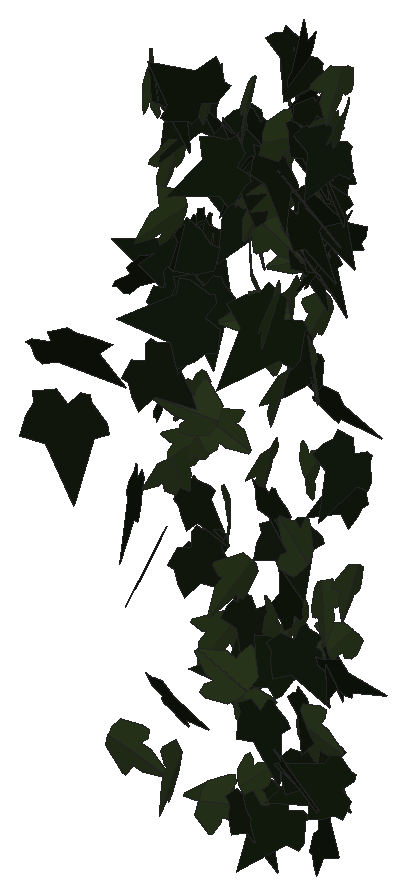
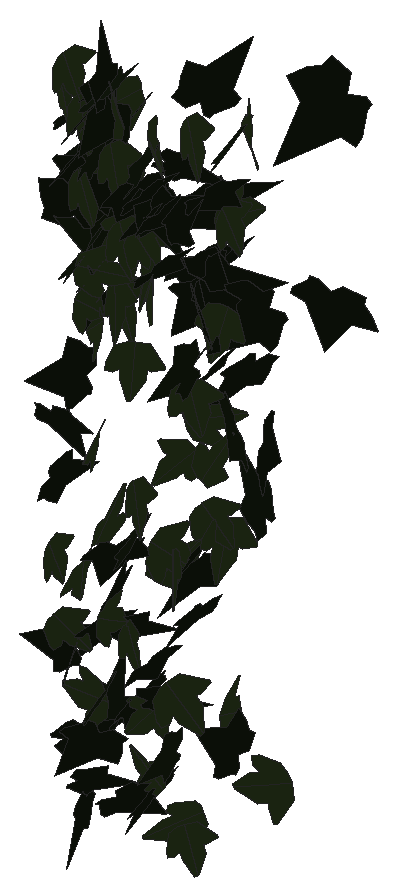
# SketchUp Ruby script. Lengths in inches.
U = 1.inch
M = Sketchup.active_model
def pt(a) = Geom::Point3d.new(a.map { |v| v * U })
def face(e, loops, mat)
  f = e.add_face(loops[0].map { |a| pt(a) })
  loops[1..].each { |l| e.add_face(l.map { |a| pt(a) }).erase! }
  f.material = f.back_material = mat if mat
  f
end
# faces: each face lists its corners as indices into pts; further lists are holes
def faces(e, pts, list, mat = nil) = list.each { |f| face(e, (f[0].is_a?(Array) ? f : [f]).map { |l| l.map { |i| pts[i] } }, mat) }
# xy, xz, yz: faces in a plane at the given z, y or x. An outline is a flat list of corners, or four numbers for a rectangle; further outlines are holes
def ring(l) = l.size == 4 ? [[l[0], l[1]], [l[2], l[1]], [l[2], l[3]], [l[0], l[3]]] : l.each_slice(2).to_a
def flat(e, list, mat, &to3) = list.each { |f| face(e, (f[0].is_a?(Array) ? f : [f]).map { |l| ring(l).map { |u, v| to3.(u, v) } }, mat) }
def xy(e, z, list, mat = nil) = flat(e, list, mat) { |x, y| [x, y, z] }
def xz(e, y, list, mat = nil) = flat(e, list, mat) { |x, z| [x, y, z] }
def yz(e, x, list, mat = nil) = flat(e, list, mat) { |y, z| [x, y, z] }
def lines(e, pts, list) = list.each { |a, b| e.add_line(pt(pts[a]), pt(pts[b])) }
# prism: a flat outline (further loops are holes) pulled along v
def prism(e, loops, v, mat = nil)
  f = face(e, loops, mat); d = Geom::Vector3d.new(v.map { |x| x * U })
  f.pushpull(f.normal.samedirection?(d) ? d.length : -d.length)
end
def box(e, o, s, mat = nil) = prism(e, [[o, [o[0] + s[0], o[1], o[2]], [o[0] + s[0], o[1] + s[1], o[2]], [o[0], o[1] + s[1], o[2]]]], [0, 0, s[2]], mat)
def at(x, y, z, deg = 0) = Geom::Transformation.translation(pt([x, y, z])) * Geom::Transformation.rotation(ORIGIN, Z_AXIS, deg.degrees)
def axes(o, x, y, z) = Geom::Transformation.new([*x, 0, *y, 0, *z, 0, *pt(o).to_a, 1])
def part(name) = M.definitions.add(name)
# library, detail: a bought-in or finely detailed component or shape, given as its bounding box
def library(name, o, s) = part(name).tap { |d| box(d.entities, o, s) }
def detail(e, o, s) = box(e.add_group.entities, o, s)
def put(e, d, t, mat = nil) = e.add_instance(d, t).tap { |i| i.material = mat if mat }
def group(e, t, mat = nil) = e.add_group.tap { |g| g.transformation = t; g.material = mat if mat }.entities
root = M.entities
M.materials.add("efeu1").color = [18, 25, 13]
M.materials.add("efeu2").color = [43, 57, 29]
c1 = part("ivyleaf_9")
p = [[1.54,2.16,1.25],[1.36,2.04,1.19],[-0.21,0.99,0.68],[-0.71,1.11,0.82],[-0.85,0.86,0.67],[-0.8,0.17,0.21],
  [-0.9,-0.01,0.1],[-0.67,-0.16,-0.02],[-0.08,-0.08,-0.05],[-0.03,-0.6,-0.4],[0.65,-0.88,-0.66],[0.83,-0.6,-0.49],
  [1.29,-0.42,-0.43],[1.8125,-0.07,-0.26],[1.21,0.44,0.15]]
faces(c1.entities,p,[[0,1,2,3,4,5,6,7,8,9,10,11,12,13,14]],"efeu1")
c2 = part("ivyleaf_10")
p = [[0,0.5,-0.03],[-0.0625,2.02,-0.43],[-0.19,2.01,-0.46],[-0.54,1.05,-0.29],[-0.52,0.625,-0.18],[-0.83,0.76,-0.28],
  [-1.16,0.64,-0.33],[-1.15,0.33,-0.24],[-0.77,-0.39,0.02],[-0.3,-0.51,0.16],[0.04,-0.48,0.23],[-0.02,2.01,-0.4375],
  [-0.06,2.01,-0.43],[0.04,-0.49,0.23],[0.67,-0.49,0.14],[1.38,0.36,-0.2],[1.375,0.51,-0.24],[0.81,0.65,-0.19],
  [0.62,0.59,-0.15],[0.6,1.09,-0.28],[0.5,1.23,-0.31]]
faces(c2.entities,p,[[0,1,2,3,4,5,6,7,8,9,10],[11,12,0,13,14,15,16,17,18,19,20]],"efeu2")
put(root,c1,axes([548.11,113.9,235.42],[1.28022,0.60227,0.19081],[0.16815,0.09079,-1.41477],[-0.60898,1.29117,0.01048]))
put(root,c1,axes([544.9,118.74,229.05],[-0.84969,-0.61122,-0.89076],[0.69545,0.55774,-1.04609],[0.82668,-1.09743,-0.03553]))
put(root,c1,axes([549.24,122.18,233.34],[-0.22968,-0.83768,-0.9062],[-0.08009,-0.9097,0.86121],[-1.23146,0.2154,0.11301]))
put(root,c1,axes([545.83,122.21,219.59],[0.02801,1.00742,0.6907],[-0.01978,-0.69042,1.00781],[1.2213,-0.03428,0.00048]))
put(root,c1,axes([545.03,123.13,223.66],[-0.22386,0.10081,-1.19076],[1.02169,-0.61225,-0.24391],[-0.61986,-1.04555,0.02801]))
put(root,c2,axes([549.99,123.5,215.83],[0.35261,0.79349,0.70985],[-0.33312,-0.628,0.86747],[1.01121,-0.48357,0.03824]))
put(root,c2,axes([546.32,124.03,210.43],[0.14476,-0.45523,1.14308],[0.69552,-0.91915,-0.45413],[1.01494,0.69481,0.14817]))
put(root,c2,axes([551.84,123.67,234.42],[0.51811,-1.04399,-0.01718],[-0.00669,0.01586,-1.16548],[1.04411,0.51816,0.00105]))
put(root,c1,axes([551.67,124.37,233.12],[-1.22341,-0.5287,0.1001],[-0.0841,-0.0577,-1.33262],[0.53148,-1.22614,0.01955]))
put(root,c1,axes([546.15,123.8125,232.875],[0.65919,-0.61663,-0.69147],[-0.23733,0.70792,-0.85755],[0.89556,0.64148,0.2817]))
put(root,c2,axes([545.22,125.4,235.57],[0.01015,-0.17762,1.12447],[0.13764,-1.11607,-0.17754],[1.13006,0.13753,0.01153]))
put(root,c2,axes([550.83,125.02,232.86],[0.24225,0.07581,-1.10045],[-1.00258,-0.4547,-0.25203],[-0.45998,1.03098,-0.03024]))
put(root,c1,axes([547.15,124.92,232.75],[-0.03803,-1.10121,-0.27767],[0.04772,0.27604,-1.10124],[1.13468,-0.04852,0.037]))
put(root,c2,axes([551.07,125.25,229.74],[0.24564,-1.1153,0.05987],[0.00144,-0.06099,-1.14197],[1.1169,0.24536,-0.0117]))
put(root,c1,axes([546.33,125.65,241.08],[0.25441,0.1856,1.10471],[-0.97872,-0.51423,0.31179],[0.54491,-1.01028,0.04424]))
put(root,c1,axes([544.4,124.68,228.46],[0.38973,-0.54202,-0.89548],[-0.18105,0.90623,-0.62732],[1.03097,0.36404,0.22835]))
put(root,c2,axes([542.2,125.73,209.32],[-0.48501,0.1138,-1.0983],[1.07896,-0.20608,-0.49782],[-0.23465,-1.18281,-0.01893]))
put(root,c2,axes([547.94,126.48,219.05],[-0.11869,-0.72826,0.86435],[0.02016,-0.87033,-0.73053],[1.13007,-0.06096,0.10381]))
put(root,c1,axes([549.83,126.25,239.08],[0.3045,-1.00657,0.18188],[0.0412,-0.17754,-1.05155],[1.02203,0.30705,-0.0118]))
put(root,c1,axes([545.73,125.98,232.6],[-0.48648,0.13082,1.16642],[-1.14777,0.21109,-0.50238],[-0.24551,-1.24605,0.03736]))
put(root,c2,axes([546.11,126.34,225.85],[0.26765,0.20594,1.03616],[-0.80324,-0.65461,0.33759],[0.68618,-0.84661,-0.00898]))
put(root,c1,axes([547.45,126.52,237.94],[-0.92473,-0.2032,0.46252],[-0.44699,-0.12042,-0.9466],[0.2354,-1.02692,0.01949]))
put(root,c1,axes([550.67,126.76,209.875],[0.89426,-0.66762,-0.15371],[0.14247,-0.066,1.11553],[-0.67011,-0.90497,0.03204]))
put(root,c2,axes([542.82,126.73,240.68],[0.22491,-0.08428,1.21566],[1.06356,-0.5898,-0.23766],[0.59478,1.08652,-0.03472]))
put(root,c1,axes([543.08,125.42,231.91],[0.63882,0.73595,0.6306],[0.39256,0.49405,-0.97426],[-0.8861,0.74944,0.02301]))
put(root,c1,axes([550.96,126.51,236.78],[0.64558,-0.77965,-0.32909],[-0.15457,0.29831,-1.00997],[0.83202,0.66037,0.06771]))
put(root,c1,axes([549.55,127.14,214.9],[-0.63647,-0.29447,0.5931],[-0.48834,-0.34687,-0.69626],[0.44723,-0.79783,0.0838]))
put(root,c1,axes([543.6875,126.87,240.48],[0.47469,-0.9316,0.0422],[0.01647,-0.03897,-1.04556],[0.93241,0.47496,-0.00301]))
put(root,c1,axes([550.82,127.38,229.99],[-0.11433,-0.75041,0.67425],[-0.14082,-0.66005,-0.75848],[0.99895,-0.17893,-0.02976]))
put(root,c1,axes([550.39,126.73,237.89],[0.85433,-0.61914,0.39765],[0.32146,-0.23407,-1.05509],[0.66191,0.91281,-0.00084]))
put(root,c1,axes([544.83,127.24,233.66],[-0.15173,0.10468,-1.0156],[0.63336,-0.79566,-0.17664],[-0.80078,-0.64915,0.05272]))
put(root,c2,axes([549.77,126.18,240.27],[-0.11552,-0.19847,-1.04461],[0.52734,0.90173,-0.22964],[0.92331,-0.53985,0.00046]))
put(root,c1,axes([544.44,127.64,229.32],[-0.09571,-0.90601,0.46397],[0.02556,-0.46801,-0.90862],[1.01758,-0.07346,0.06647]))
put(root,c1,axes([545.39,126.47,219.18],[0.36268,-0.51266,-0.89681],[-0.186,0.90254,-0.59115],[1.01612,0.34819,0.21189]))
put(root,c1,axes([548.39,127.19,212.17],[0.28537,-1.01097,-0.18089],[-0.05662,0.17197,-1.05044],[1.02546,0.29083,-0.00766]))
put(root,c1,axes([543.23,127.26,211.11],[0.49177,-0.46473,0.78965],[0.62213,-0.48859,-0.67498],[0.67267,0.79163,0.04698]))
put(root,c2,axes([543.57,127.42,237.01],[0.04502,-0.94848,0.37058],[0.13585,-0.36203,-0.94311],[1.0092,0.09105,0.11042]))
put(root,c1,axes([544.14,126.21,226.11],[-0.0895,0.57934,1.11363],[-0.18649,1.09793,-0.58616],[-1.24138,-0.20671,0.00777]))
put(root,c1,axes([547.66,127.22,207.77],[0.47472,-0.93415,-0.35024],[-0.13461,0.32435,-1.04754],[0.98853,0.49278,0.02555]))
put(root,c1,axes([550.39,127.49,240.21],[0.48792,-0.87105,-0.11834],[-0.07118,0.09576,-0.99828],[0.87616,0.49285,-0.0152]))
put(root,c2,axes([550.41,127.7,229.7],[-0.47713,0.53739,-0.87193],[0.52184,-0.70014,-0.71707],[-0.88132,-0.70549,0.04747]))
put(root,c1,axes([551.43,128.08,239.78],[-0.3104,-0.90416,0.41479],[-0.04839,-0.42027,-0.95233],[0.99358,-0.30293,0.0832]))
put(root,c1,axes([548.93,128.07,207.33],[-0.70046,-0.81117,0.30777],[-0.18438,-0.24734,-1.07154],[0.84778,-0.72401,0.02124]))
put(root,c1,axes([549.87,127.64,234.5],[0.6541,-0.61005,0.54218],[0.38555,-0.38144,-0.89432],[0.71935,0.75915,-0.01367]))
put(root,c2,axes([547.38,127.57,208.42],[0.57559,-0.17565,-0.67433],[0.64036,-0.21157,0.60171],[-0.27478,-0.86097,-0.01029]))
put(root,c1,axes([544.59,127.36,221.12],[0.52327,-0.6204,-0.48779],[-0.18249,0.4743,-0.79899],[0.76781,0.53554,0.14254]))
put(root,c1,axes([543.99,127.74,231.3],[0.53555,-0.9246,-0.15239],[-0.06095,0.14079,-1.06836],[0.93509,0.53872,0.01765]))
put(root,c2,axes([545.32,127.71,240.76],[0.14923,-1.08152,-0.05502],[-0.00686,0.05459,-1.09177],[1.0829,0.14939,0.00066]))
put(root,c1,axes([544.5,127.57,233.1],[-0.271,-0.50327,-0.93319],[0.51722,0.77806,-0.56981],[0.92553,-0.58216,0.04518]))
put(root,c1,axes([551.67,128.23,209.31],[-0.39258,-0.77052,-0.50341],[-0.21501,-0.45537,0.86467],[-0.89492,0.44741,0.01309]))
put(root,c2,axes([545.73,127.2,207.08],[-0.14319,-0.3257,-1.00644],[0.76737,0.66708,-0.32506],[0.72812,-0.76709,0.14465]))
put(root,c2,axes([543.67,127.65,232.23],[-1.01831,0.00515,-0.09705],[0.09704,-0.00231,-1.01832],[-0.00535,-1.02292,0.00181]))
put(root,c2,axes([549.79,128,219.84],[-0.24524,1.02137,0.39064],[0.06949,-0.38497,1.0502],[1.09132,0.25404,0.02091]))
put(root,c2,axes([543.89,128.45,225.13],[-0.20392,-0.51942,-0.76545],[-0.30548,-0.70205,0.55778],[-0.87315,0.36693,-0.01637]))
put(root,c2,axes([543.41,127.68,222.04],[-0.40268,-0.98545,-0.34394],[0.12908,0.3188,-1.06455],[1.03573,-0.42286,-0.00104]))
put(root,c2,axes([550.1,128.12,211.75],[-0.16467,0.10605,-1.11198],[1.00427,-0.47807,-0.19431],[-0.48907,-1.01739,-0.02461]))
put(root,c2,axes([548.55,127.68,234.85],[-0.67035,-0.33147,-0.64256],[0.62083,0.18523,-0.74323],[0.37058,-0.90991,0.08278]))
put(root,c2,axes([547.25,127.83,212.0625],[-0.69725,-0.07575,-0.56826],[0.57195,-0.03088,-0.69767],[0.0391,-0.89896,0.07185]))
put(root,c1,axes([550.34,128.47,237.6],[0.69213,-0.80626,0.01305],[0.00159,0.01856,1.06251],[-0.80636,-0.692,0.01329]))
put(root,c2,axes([545.71,127.45,224.75],[0.47264,0.38009,0.74129],[0.39346,0.64938,-0.58383],[-0.73428,0.59262,0.16431]))
put(root,c2,axes([547.8125,127.4,232.76],[-0.5379,0.34428,0.90384],[-0.75066,0.50355,-0.63855],[-0.60989,-0.92342,-0.01122]))
put(root,c1,axes([549.57,127.96,215.6],[0.20653,-0.86307,-0.53471],[0.0846,0.5584,-0.86862],[1.01175,0.12949,0.18179]))
put(root,c1,axes([551.13,128.34,235.1],[0.93791,-0.05542,0.63483],[-0.63456,0.02244,0.93946],[-0.05848,-1.13233,-0.01245]))
put(root,c2,axes([543.87,128.375,223.02],[-0.51478,-0.59187,0.52175],[-0.29196,-0.43587,-0.7825],[0.733,-0.58927,0.05475]))
put(root,c2,axes([545.16,128.21,206.86],[-0.56038,-0.65111,0.2249],[-0.14844,-0.16897,-0.85905],[0.67267,-0.57971,-0.00221]))
put(root,c1,axes([550.66,128.1,236.96],[-0.35944,-0.27514,-1.03314],[0.82778,0.61821,-0.45263],[0.67666,-0.90244,0.00492]))
put(root,c1,axes([543.59,128.84,238.73],[-0.5246,-0.89633,0.25874],[-0.12115,-0.22887,-1.03851],[0.92503,-0.5383,0.01072]))
put(root,c1,axes([552.11,128.53,225.04],[-0.97667,-0.30246,-0.28557],[0.27211,0.08665,-1.02243],[0.31462,-1.01386,-0.00219]))
put(root,c1,axes([549.59,128.88,211.83],[0.04437,-0.68309,0.67983],[0.09691,-0.67394,-0.68349],[0.95885,0.09973,0.03763]))
put(root,c2,axes([550.73,128.34,240.29],[-0.09986,-1.03888,0.04189],[0.0035,-0.04242,-1.04364],[1.03972,-0.09963,0.00754]))
put(root,c1,axes([546.82,128.57,213],[-0.5943,0.04,0.67268],[-0.66715,-0.1613,-0.57982],[0.09495,-0.88299,0.13639]))
put(root,c1,axes([549.28,128.125,216.85],[-0.13518,-0.68569,0.59126],[0.12202,0.57856,0.69886],[-0.89715,0.18201,0.00596]))
put(root,c2,axes([549.03,128.15,231.77],[0.09846,-0.9927,-0.27687],[0.02444,0.2803,-0.99631],[1.0303,0.08821,0.05009]))
put(root,c2,axes([550.22,128.93,231.24],[-0.00368,-0.60279,0.81926],[0.30101,-0.78321,-0.57491],[0.97156,0.24038,0.18122]))
put(root,c2,axes([550.63,128.46,236.76],[-0.05469,-1.02546,0.1331],[-0.01065,-0.13272,-1.02691],[1.034,-0.05561,-0.00354]))
put(root,c1,axes([550.59,127.61,233.375],[-0.48459,1.0072,-0.10852],[-0.06711,0.08812,1.11749],[1.01081,0.48871,0.02216]))
put(root,c1,axes([546.95,128.4,237.28],[-0.49463,0.78891,-0.58113],[0.30039,-0.49754,-0.93112],[-0.93266,-0.57864,0.00831]))
put(root,c2,axes([551.77,128.34,241.11],[0.34298,-0.93518,-0.14007],[-0.05257,0.12991,-0.99608],[0.94415,0.34695,-0.00458]))
put(root,c2,axes([548.9375,129.01,216.35],[-0.01164,-0.42153,0.86806],[0.30877,-0.82411,-0.39604],[0.91427,0.27296,0.1448]))
put(root,c1,axes([544.41,128.2,218.14],[0.38125,-0.682,-0.51529],[-0.07502,0.53534,-0.76406],[0.85148,0.35253,0.1634]))
put(root,c2,axes([546.45,128.86,240.2],[0.65956,-0.7004,0.64569],[0.44694,-0.46603,-0.96206],[0.84126,0.79672,0.00489]))
put(root,c2,axes([550.66,128.46,218.06],[-0.10053,1.00304,-0.28661],[0.03221,-0.28482,-1.00806],[-1.04269,-0.10551,-0.0035]))
put(root,c1,axes([544.16,128.72,233.14],[-0.6361,0.10357,-0.85726],[0.84738,-0.12983,-0.64446],[-0.16601,-1.05956,-0.00482]))
put(root,c2,axes([547.95,128.35,229.29],[-0.85831,-0.51145,-0.00686],[0.00625,0.00291,-0.99914],[0.51146,-0.85833,0.0007]))
put(root,c2,axes([550.41,127.67,224.04],[0.21686,0.00371,-0.98074],[-0.15009,0.99272,-0.02944],[0.96919,0.15291,0.21488]))
put(root,c1,axes([547.05,128.875,238.78],[0.47247,-0.85734,0.3624],[0.14523,-0.33353,-0.9784],[0.91939,0.49327,-0.03168]))
put(root,c1,axes([550.64,128.39,227.35],[0.84374,-0.27506,0.55498],[0.51748,-0.20238,-0.88703],[0.3404,0.98942,-0.02715]))
put(root,c2,axes([551.15,128.82,242.51],[-0.16023,-0.92843,0.35833],[0.15766,-0.38205,-0.91937],[0.98261,-0.0901,0.20594]))
put(root,c1,axes([546.09,129.29,234.41],[-0.3928,-0.89701,0.42334],[-0.04369,-0.43924,-0.97124],[0.99093,-0.37494,0.12499]))
put(root,c2,axes([547.18,128.9375,235.4375],[-0.10024,-0.90204,0.4628],[-0.00835,-0.4643,-0.90678],[1.0138,-0.09301,0.03829]))
put(root,c1,axes([546.7,128.96,236.62],[0.00532,-1.01861,-0.0839],[0.00639,0.08393,-1.0186],[1.02204,0.00477,0.0068]))
put(root,c1,axes([549.89,128.35,210.16],[-0.0959,-0.48991,-0.89341],[0.33732,0.8315,-0.49217],[0.96147,-0.34058,0.08356]))
put(root,c1,axes([549.83,129.03,240.68],[0.36458,-1.0688,0.09804],[0.02725,-0.09429,-1.12926],[1.07294,0.36557,-0.00463]))
put(root,c1,axes([550.93,128.65,214.21],[0.55307,-0.19838,0.69335],[0.6612,-0.20934,-0.58733],[0.28791,0.86185,0.01693]))
put(root,c1,axes([549.42,127.81,240.67],[0.26189,0.88766,0.62906],[0.18335,0.60177,-0.92548],[-1.0724,0.31966,-0.00461]))
put(root,c2,axes([548.66,128.8125,238.85],[-0.09909,-1.0426,0.00152],[-0.0004,-0.00149,-1.0473],[1.0426,-0.09909,-0.00026]))
put(root,c1,axes([550.57,129.16,238.2],[0.27395,-0.94111,0.13728],[0.03401,-0.13307,-0.98016],[0.95046,0.27601,-0.00449]))
put(root,c1,axes([549,128.89,241.92],[-0.03105,0.78078,0.7162],[-0.25872,-0.70041,0.75234],[1.02744,-0.15277,0.21109]))
put(root,c1,axes([548.44,128.93,220.01],[-0.18763,-0.85694,-0.49129],[0.16338,0.46627,-0.87568],[0.97418,-0.24324,0.05224]))
put(root,c2,axes([549.66,129.27,233.21],[-0.17558,-0.04246,1.0018],[-0.66558,-0.75573,-0.14868],[0.74994,-0.68066,0.10259]))
put(root,c1,axes([549.96,129.02,233.9],[0.56357,-0.89168,-0.02546],[-0.01357,0.02154,-1.05485],[0.89194,0.56373,0.00004]))
put(root,c2,axes([545.03,129.25,214.22],[-0.48675,-0.77642,0.61795],[-0.27934,-0.55324,-0.91516],[0.95219,-0.55921,0.04741]))
put(root,c2,axes([548.06,128.58,215.74],[-0.5497,0.19791,0.69322],[-0.67829,0.15335,-0.58164],[-0.24423,-0.87133,0.0551]))
put(root,c1,axes([546.31,129.38,215.28],[-0.10717,-0.96755,0.14437],[-0.01579,-0.1435,-0.97346],[0.97813,-0.10832,0.0001]))
put(root,c2,axes([551.56,129.26,218.87],[0.07665,-0.86137,0.41055],[0.23566,-0.38203,-0.84552],[0.92465,0.16877,0.18146]))
put(root,c1,axes([545.74,128.77,236.61],[0.23071,-0.18701,0.99494],[-0.7539,0.64931,0.29686],[-0.67565,-0.78837,0.00849]))
put(root,c1,axes([551.24,129.65,222.74],[0.03862,-0.40126,-0.83176],[0.32508,-0.77329,0.38814],[-0.86438,-0.30876,0.10882]))
put(root,c1,axes([548.55,129.79,242.18],[-0.2824,-0.87158,0.69569],[0.20377,-0.7459,-0.85177],[1.09642,-0.08586,0.33749]))
put(root,c1,axes([549.9,129.47,208.41],[-0.64066,-0.27348,0.56649],[-0.47257,-0.32443,-0.69106],[0.41519,-0.79126,0.08756]))
put(root,c1,axes([545.63,129.45,237.41],[-0.08426,-0.99949,0.10595],[-0.00714,-0.10573,-1.00304],[1.00507,-0.08454,0.00175]))
put(root,c2,axes([544.31,129.05,228.98],[-0.69192,-0.60066,0.27656],[-0.19873,-0.19289,-0.91615],[0.6307,-0.71975,0.01473]))
put(root,c1,axes([550.27,129.59,214.39],[0.34543,-0.26956,-0.91918],[0.80699,-0.44453,0.43363],[-0.51606,-0.87556,0.06282]))
put(root,c1,axes([549.08,129.13,233.65],[0.475,-0.85088,-0.08182],[-0.03385,0.07481,-0.97446],[0.85414,0.47615,0.00688]))
put(root,c1,axes([546.41,129.71,238.11],[-0.2919,-0.91853,0.38644],[-0.02618,-0.39547,-0.95977],[0.99617,-0.27954,0.08801]))
put(root,c1,axes([547.2,129.11,238.01],[-0.01832,-1.00316,-0.469],[-0.0106,0.4692,-1.00318],[1.10733,-0.0121,-0.01736]))
put(root,c1,axes([544.43,128.85,230.12],[0.90215,-0.32944,0.02387],[0.02188,-0.00967,-0.96042],[0.32958,0.90242,-0.00158]))
put(root,c1,axes([550.4375,128.47,206.76],[0.2663,-0.22295,-0.94817],[-0.76329,0.56287,-0.34672],[0.60508,0.80816,-0.02009]))
put(root,c2,axes([547.84,129.17,235.53],[-0.18682,-1.01144,0.11178],[-0.00413,-0.1129,-1.02842],[1.01759,-0.18615,0.01635]))
put(root,c1,axes([547.11,129.34,221.04],[0.51614,-0.85421,0.16966],[0.06625,-0.15814,-0.99773],[0.86837,0.51978,-0.02473]))
put(root,c2,axes([547.77,129.57,241.32],[0.12712,-0.18077,-1.02809],[0.60557,-0.83082,0.22096],[-0.85025,-0.61876,0.00367]))
put(root,c2,axes([545.37,128.72,220.29],[0.5902,-0.60662,-0.52893],[-0.12912,0.57604,-0.80473],[0.7944,0.54431,0.26217]))
put(root,c2,axes([546.61,128.94,233.91],[-0.62373,0.74173,-0.10148],[0.05824,-0.08361,-0.96908],[-0.74637,-0.62638,0.00918]))
put(root,c2,axes([547.2,129.09,223.15],[0.10571,-0.97124,-0.12365],[-0.00896,0.1234,-0.97696],[0.97903,0.106,0.00441]))
put(root,c2,axes([550.96,129.48,215.7],[-0.45539,-0.45054,0.6455],[-0.33739,-0.56205,-0.63032],[0.71122,-0.55511,0.1143]))
put(root,c1,axes([545.21,129.02,211.24],[0.77308,-0.4333,-0.04863],[-0.03451,0.03787,-0.88608],[0.43465,0.77368,0.01614]))
